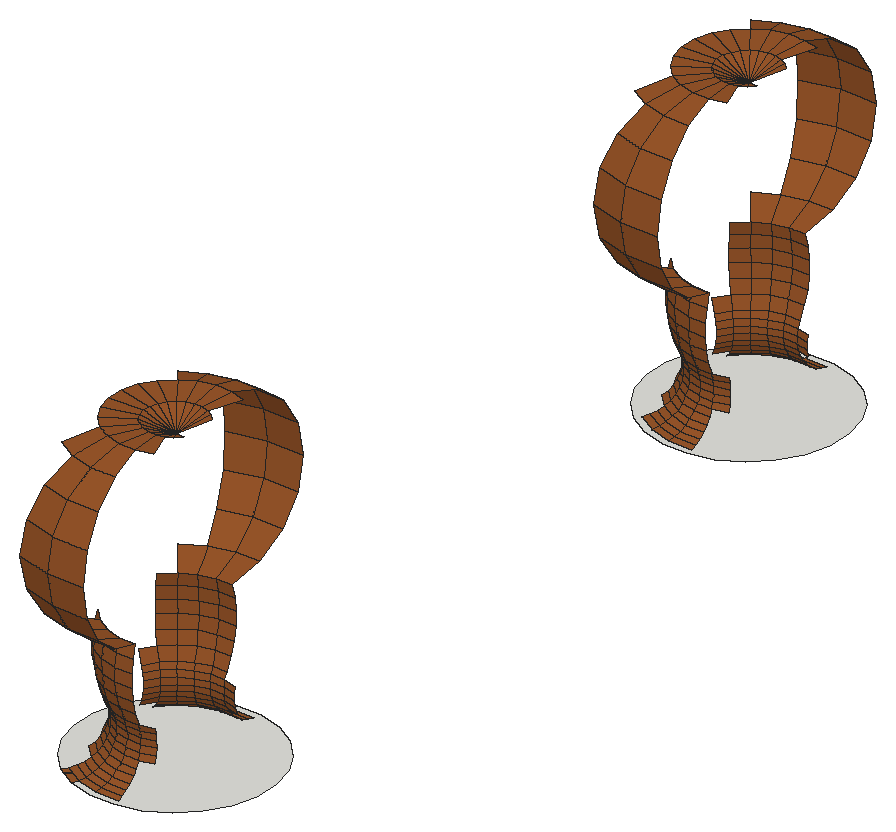
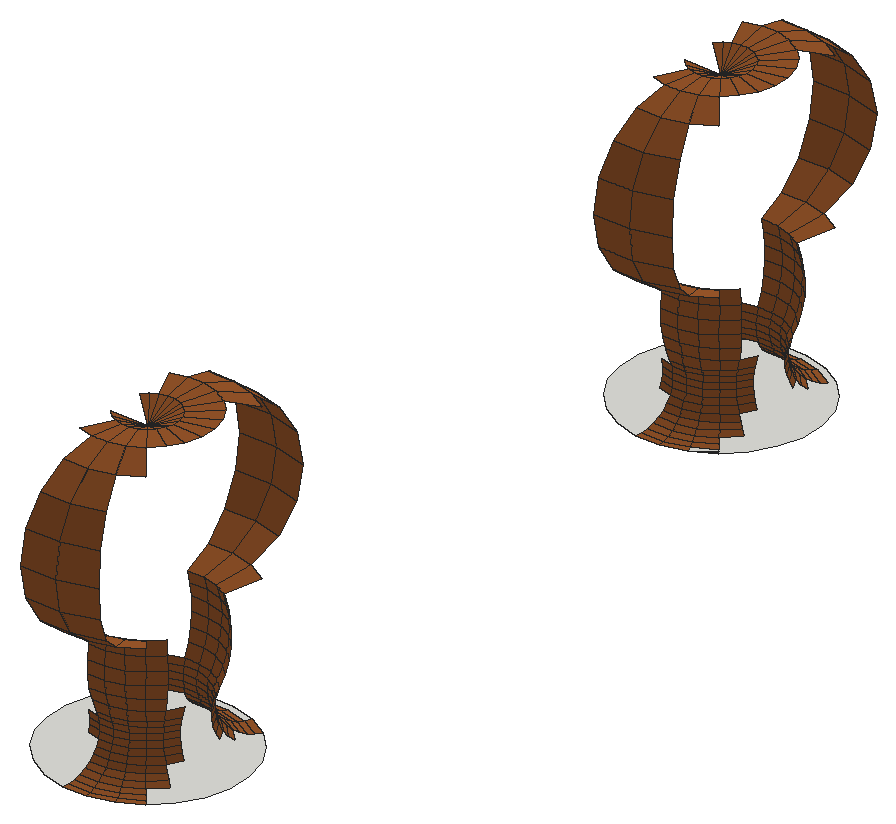
# SketchUp Ruby script. Lengths in inches.
U = 1.inch
M = Sketchup.active_model
def pt(a) = Geom::Point3d.new(a.map { |v| v * U })
def face(e, loops, mat)
  f = e.add_face(loops[0].map { |a| pt(a) })
  loops[1..].each { |l| e.add_face(l.map { |a| pt(a) }).erase! }
  f.material = f.back_material = mat if mat
  f
end
# faces: each face lists its corners as indices into pts; further lists are holes
def faces(e, pts, list, mat = nil) = list.each { |f| face(e, (f[0].is_a?(Array) ? f : [f]).map { |l| l.map { |i| pts[i] } }, mat) }
# xy, xz, yz: faces in a plane at the given z, y or x. An outline is a flat list of corners, or four numbers for a rectangle; further outlines are holes
def ring(l) = l.size == 4 ? [[l[0], l[1]], [l[2], l[1]], [l[2], l[3]], [l[0], l[3]]] : l.each_slice(2).to_a
def flat(e, list, mat, &to3) = list.each { |f| face(e, (f[0].is_a?(Array) ? f : [f]).map { |l| ring(l).map { |u, v| to3.(u, v) } }, mat) }
def xy(e, z, list, mat = nil) = flat(e, list, mat) { |x, y| [x, y, z] }
def xz(e, y, list, mat = nil) = flat(e, list, mat) { |x, z| [x, y, z] }
def yz(e, x, list, mat = nil) = flat(e, list, mat) { |y, z| [x, y, z] }
def lines(e, pts, list) = list.each { |a, b| e.add_line(pt(pts[a]), pt(pts[b])) }
# prism: a flat outline (further loops are holes) pulled along v
def prism(e, loops, v, mat = nil)
  f = face(e, loops, mat); d = Geom::Vector3d.new(v.map { |x| x * U })
  f.pushpull(f.normal.samedirection?(d) ? d.length : -d.length)
end
def box(e, o, s, mat = nil) = prism(e, [[o, [o[0] + s[0], o[1], o[2]], [o[0] + s[0], o[1] + s[1], o[2]], [o[0], o[1] + s[1], o[2]]]], [0, 0, s[2]], mat)
def at(x, y, z, deg = 0) = Geom::Transformation.translation(pt([x, y, z])) * Geom::Transformation.rotation(ORIGIN, Z_AXIS, deg.degrees)
def axes(o, x, y, z) = Geom::Transformation.new([*x, 0, *y, 0, *z, 0, *pt(o).to_a, 1])
def part(name) = M.definitions.add(name)
# library, detail: a bought-in or finely detailed component or shape, given as its bounding box
def library(name, o, s) = part(name).tap { |d| box(d.entities, o, s) }
def detail(e, o, s) = box(e.add_group.entities, o, s)
def put(e, d, t, mat = nil) = e.add_instance(d, t).tap { |i| i.material = mat if mat }
def group(e, t, mat = nil) = e.add_group.tap { |g| g.transformation = t; g.material = mat if mat }.entities
root = M.entities
M.materials.add("[Wood Cherry Original]").color = [152, 86, 42]
xy(root,6,[[160.74,47.97,161.3,47.97,161.84,48.11,162.32,48.39,162.72,48.78,163,49.26,163.15,49.8,163.15,50.36,163.01,50.9,162.73,51.38,162.34,51.78,161.85,52.06,161.32,52.21,160.76,52.21,160.22,52.07,159.73,51.79,159.34,51.4,159.06,50.91,158.91,50.375,158.91,49.82,159.05,49.28,159.33,48.79,159.72,48.4,160.2,48.11],[160.74,64.59,161.3,64.59,161.84,64.73,162.32,65.01,162.72,65.4,163,65.89,163.15,66.42,163.15,66.98,163.01,67.52,162.73,68.01,162.34,68.4,161.85,68.69,161.32,68.83,160.76,68.83,160.22,68.69,159.73,68.41,159.34,68.02,159.06,67.54,158.91,67,158.91,66.44,159.05,65.9,159.33,65.42,159.72,65.02,160.2,64.74]])
xy(root,6,[[160.74,47.97,160.76,48.12,160.26,48.25,160.2,48.11],[160.74,47.97,161.3,47.97,161.28,48.12,160.76,48.12],[160.2,48.11,160.26,48.25,159.8125,48.51,159.72,48.4],[159.82,51.67,160.27,51.93,160.22,52.07,159.73,51.79],[160.27,51.93,160.78,52.06,160.76,52.21,160.22,52.07],
  [160.78,52.06,161.3,52.06,161.32,52.21,160.76,52.21],[160.74,64.59,160.76,64.74,160.26,64.88,160.2,64.74],[160.74,64.59,161.3,64.59,161.28,64.74,160.76,64.74],[160.2,64.74,160.26,64.88,159.8125,65.14,159.72,65.02],[159.82,68.29,160.27,68.55,160.22,68.69,159.73,68.41],
  [160.27,68.55,160.78,68.68,160.76,68.83,160.22,68.69],[160.78,68.68,161.3,68.68,161.32,68.83,160.76,68.83]],"[Wood Cherry Original]")
xz(root,48.59,[[160.83,8.1,161.22,8.4]],"[Wood Cherry Original]")
xz(root,51.28,[[160.875,6.79,161.19,6.94]],"[Wood Cherry Original]")
xz(root,65.52,[[160.87,6.79,161.18,6.94]],"[Wood Cherry Original]")
xz(root,67.9,[[160.875,6.79,161.19,6.94]],"[Wood Cherry Original]")
xz(root,68.21,[[160.84,8.1,161.23,8.4]],"[Wood Cherry Original]")
p = [[160.32,48.39,6.03],[160.26,48.25,6],[160.76,48.12,6],[160.78,48.27,6.03],[161.28,48.12,6],[161.26,48.26,6.03],
  [159.9,48.63,6.03],[159.8125,48.51,6],[160.37,48.52,6.08],[160.8,48.41,6.08],[161.24,48.4,6.08],[159.99,48.75,6.08],
  [160.38,51.66,6.08],[160.33,51.79,6.03],[159.91,51.55,6.03],[160,51.4375,6.08],[160.27,51.93,6],[159.82,51.67,6],
  [160.8125,51.77,6.08],[160.8,51.91,6.03],[160.78,52.06,6],[161.26,51.77,6.08],[161.28,51.91,6.03],[161.3,52.06,6],
  [160.32,65.02,6.03],[160.26,64.88,6],[160.76,64.74,6],[160.78,64.89,6.03],[161.28,64.74,6],[161.26,64.89,6.03],
  [159.9,65.26,6.03],[159.8125,65.14,6],[160.37,65.15,6.08],[160.8,65.03,6.08],[161.24,65.03,6.08],[159.99,65.37,6.08],
  [160.38,68.28,6.08],[160.33,68.41,6.03],[159.91,68.18,6.03],[160,68.0625,6.08],[160.27,68.55,6],[159.82,68.29,6],
  [160.8125,68.4,6.08],[160.8,68.54,6.03],[160.78,68.68,6],[161.26,68.39,6.08],[161.28,68.53,6.03],[161.3,68.68,6],
  [160.42,48.64,6.16],[160.82,48.54,6.16],[161.23,48.53,6.16],[160.07,48.85,6.16],[160.08,51.33,6.16],[159.6875,51.125,6.08],
  [159.79,51.05,6.16],[160.43,51.54,6.16],[160.83,51.64,6.16],[161.24,51.64,6.16],[160.42,65.27,6.16],[160.82,65.16,6.16],
  [161.23,65.16,6.16],[160.07,65.47,6.16],[160.08,67.96,6.16],[159.6875,67.75,6.08],[159.79,67.67,6.16],[160.43,68.16,6.16],
  [160.83,68.27,6.16],[161.24,68.26,6.16],[160.47,48.75,6.25],[160.83,48.65,6.25],[161.21,48.65,6.25],[160.14,48.94,6.25],
  [159.875,49.21,6.25],[159.78,49.14,6.16],[160.15,51.24,6.25],[159.88,50.97,6.25],[160.48,51.43,6.25],[160.84,51.53,6.25],
  [161.22,51.52,6.25],[160.47,65.375,6.25],[160.83,65.27,6.25],[161.21,65.27,6.25],[160.14,65.56,6.25],[159.875,65.83,6.25],
  [159.78,65.76,6.16],[160.15,67.87,6.25],[159.88,67.6,6.25],[160.48,68.05,6.25],[160.84,68.15,6.25],[161.22,68.15,6.25],
  [160.51,48.84,6.37],[160.85,48.75,6.37],[161.2,48.74,6.37],[160.2,49.02,6.37],[159.95,49.27,6.37],[160.21,51.16,6.37],
  [159.96,50.92,6.37],[160.51,51.34,6.37],[160.86,51.43,6.37],[161.21,51.43,6.37],[160.51,65.46,6.37],[160.85,65.37,6.37],
  [161.2,65.37,6.37],[160.2,65.64,6.37],[159.95,65.89,6.37],[160.21,67.79,6.37],[159.96,67.54,6.37],[160.51,67.97,6.37],
  [160.86,68.06,6.37],[161.21,68.05,6.37],[160.53,48.91,6.5],[160.86,48.82,6.5],[161.19,48.82,6.5],[160.25,49.08,6.5],
  [160.01,49.3125,6.5],[159.84,49.6,6.5],[159.78,49.57,6.37],[160.02,50.87,6.5],[159.78,50.61,6.37],[159.85,50.58,6.5],
  [160.25,51.1,6.5],[160.54,51.27,6.5],[160.87,51.36,6.5],[161.2,51.35,6.5],[160.53,65.53,6.5],[160.86,65.44,6.5],
  [161.19,65.44,6.5],[160.25,65.7,6.5],[160.01,65.9375,6.5],[159.84,66.23,6.5],[159.78,66.2,6.37],[160.02,67.49,6.5],
  [159.78,67.24,6.37],[159.85,67.21,6.5],[160.25,67.73,6.5],[160.54,67.9,6.5],[160.87,67.98,6.5],[161.2,67.98,6.5],
  [160.55,48.95,6.64],[160.86,48.87,6.64],[161.18,48.87,6.64],[161.51,48.9,6.5],[161.49,48.95,6.64],[160.28,49.12,6.64],
  [160.05,49.34,6.64],[159.89,49.62,6.64],[160.06,50.84,6.64],[159.9,50.5625,6.64],[160.28,51.0625,6.64],[160.5625,51.22,6.64],
  [160.87,51.3,6.64],[161.5,51.22,6.64],[161.52,51.27,6.5],[161.19,51.3,6.64],[160.55,65.58,6.64],[160.86,65.5,6.64],
  [161.18,65.49,6.64],[161.51,65.53,6.5],[161.49,65.58,6.64],[160.28,65.74,6.64],[160.05,65.97,6.64],[159.89,66.25,6.64],
  [160.06,67.46,6.64],[159.9,67.1875,6.64],[160.28,67.6875,6.64],[160.5625,67.85,6.64],[160.87,67.93,6.64],[161.19,67.93,6.64],
  [160.5625,48.98,6.79],[160.87,48.9,6.79],[161.18,48.9,6.79],[161.48,48.98,6.79],[160.29,49.14,6.79],[160.07,49.36,6.79],
  [159.92,49.63,6.79],[160.08,50.82,6.79],[159.92,50.55,6.79],[160.3,51.04,6.79],[160.57,51.2,6.79],[160.875,51.28,6.79],
  [161.49,51.2,6.79],[161.19,51.28,6.79],[160.5625,65.6,6.79],[160.87,65.52,6.79],[161.18,65.52,6.79],[161.48,65.6,6.79],
  [160.29,65.76,6.79],[160.07,65.98,6.79],[159.92,66.26,6.79],[160.08,67.45,6.79],[159.92,67.18,6.79],[160.3,67.67,6.79],
  [160.57,67.82,6.79],[160.875,67.9,6.79],[161.49,67.82,6.79],[161.5,67.84,6.64],[161.19,67.9,6.79],[160.5625,48.98,6.94],
  [160.87,48.9,6.94],[161.18,48.89,6.94],[161.48,48.97,6.94],[160.29,49.14,6.94],[160.07,49.36,6.94],[159.92,49.63,6.94],
  [160.08,50.82,6.94],[159.92,50.55,6.94],[160.3,51.04,6.94],[160.57,51.2,6.94],[160.875,51.28,6.94],[161.49,51.2,6.94],
  [161.19,51.28,6.94],[160.5625,65.6,6.94],[160.87,65.52,6.94],[161.18,65.52,6.94],[161.48,65.6,6.94],[160.29,65.76,6.94],
  [160.07,65.98,6.94],[159.92,66.26,6.94],[160.08,67.45,6.94],[159.92,67.18,6.94],[160.3,67.67,6.94],[160.57,67.82,6.94],
  [160.875,67.9,6.94],[161.49,67.82,6.94],[161.19,67.9,6.94],[160.55,48.95,7.09],[160.86,48.87,7.09],[161.18,48.87,7.09],
  [161.49,48.95,7.09],[160.28,49.12,7.09],[160.05,49.34,7.09],[159.89,49.62,7.09],[160.06,50.84,7.09],[159.89,50.5625,7.09],
  [160.28,51.06,7.09],[160.5625,51.22,7.09],[160.87,51.31,7.09],[161.5,51.22,7.09],[161.19,51.3,7.09],[160.55,65.58,7.09],
  [160.86,65.49,7.09],[161.18,65.49,7.09],[161.49,65.58,7.09],[160.28,65.74,7.09],[160.05,65.97,7.09],[159.89,66.25,7.09],
  [160.06,67.46,7.09],[159.89,67.1875,7.09],[160.28,67.69,7.09],[160.5625,67.85,7.09],[160.87,67.93,7.09],[161.5,67.85,7.09],
  [161.19,67.93,7.09],[160.53,48.91,7.23],[160.86,48.82,7.23],[161.19,48.82,7.23],[161.51,48.9,7.23],[160.24,49.07,7.23],
  [160.01,49.3125,7.23],[159.84,49.6,7.23],[160.02,50.87,7.23],[159.85,50.58,7.23],[160.25,51.11,7.23],[160.54,51.27,7.23],
  [160.87,51.36,7.23],[161.2,51.36,7.23],[160.53,65.53,7.23],[160.86,65.44,7.23],[161.19,65.44,7.23],[161.51,65.53,7.23],
  [160.24,65.7,7.23],[160.01,65.9375,7.23],[159.84,66.23,7.23],[160.02,67.5,7.23],[159.85,67.21,7.23],[160.25,67.73,7.23],
  [160.54,67.9,7.23],[160.87,67.98,7.23],[161.2,67.98,7.23],[160.49,48.8,7.51],[160.84,48.71,7.51],[161.2,48.71,7.51],
  [160.18,48.99,7.51],[159.92,49.24,7.51],[159.93,50.9375,7.51],[159.74,50.625,7.51],[160.19,51.19,7.51],[160.5,51.375,7.51],
  [160.85,51.47,7.51],[161.22,51.47,7.51],[160.49,65.43,7.51],[160.84,65.33,7.51],[161.2,65.33,7.51],[160.18,65.61,7.51],
  [159.92,65.87,7.51],[159.93,67.5625,7.51],[159.74,67.25,7.51],[160.19,67.82,7.51],[160.5,68,7.51],[160.85,68.09,7.51],
  [161.22,68.09,7.51],[160.46,48.73,7.8],[160.83,48.63,7.8],[161.21,48.63,7.8],[160.13,48.93,7.8],[159.86,49.2,7.8],
  [160.14,51.25,7.8],[159.87,50.98,7.8],[160.47,51.45,7.8],[160.84,51.54,7.8],[161.23,51.54,7.8],[160.46,65.36,7.8],
  [160.83,65.26,7.8],[161.21,65.26,7.8],[160.13,65.55,7.8],[159.86,65.82,7.8],[160.14,67.88,7.8],[159.87,67.61,7.8],
  [160.47,68.07,7.8],[160.84,68.17,7.8],[161.23,68.17,7.8],[160.45,48.7,8.1],[160.83,48.59,8.1],[161.22,48.59,8.1],
  [160.11,48.89,8.1],[159.83,49.17,8.1],[160.12,51.29,8.1],[159.84,51.01,8.1],[160.46,51.48,8.1],[160.84,51.58,8.1],
  [161.23,51.58,8.1],[160.45,65.32,8.1],[160.83,65.22,8.1],[161.22,65.22,8.1],[160.11,65.52,8.1],[159.83,65.8,8.1],
  [160.12,67.91,8.1],[159.84,67.63,8.1],[160.46,68.11,8.1],[160.84,68.21,8.1],[161.23,68.21,8.1],[160.44,48.69,8.4],
  [160.83,48.59,8.4],[160.1,48.89,8.4],[159.83,49.17,8.4],[160.11,51.29,8.4],[159.83,51.01,8.4],[160.46,51.48,8.4],
  [160.84,51.59,8.4],[161.23,51.58,8.4],[160.44,65.32,8.4],[160.83,65.22,8.4],[161.22,65.21,8.4],[160.1,65.52,8.4],
  [159.83,65.8,8.4],[160.11,67.91,8.4],[159.83,67.64,8.4],[160.46,68.11,8.4],[160.84,68.21,8.4],[160.46,48.73,8.7],
  [160.83,48.625,8.7],[161.22,48.59,8.4],[161.22,48.62,8.7],[160.125,48.92,8.7],[159.85,49.19,8.7],[160.13,51.26,8.7],
  [159.86,50.99,8.7],[160.47,51.45,8.7],[160.84,51.55,8.7],[161.23,51.55,8.7],[160.46,65.35,8.7],[160.83,65.25,8.7],
  [161.22,65.25,8.7],[160.125,65.54,8.7],[159.85,65.82,8.7],[160.13,67.89,8.7],[159.86,67.62,8.7],[160.47,68.08,8.7],
  [160.84,68.18,8.7],[161.23,68.17,8.7],[161.23,68.21,8.4],[160.49,48.79,8.99],[160.84,48.69,8.99],[161.21,48.69,8.99],
  [160.17,48.98,8.99],[159.91,49.24,8.99],[160.18,51.21,8.99],[159.92,50.95,8.99],[160.5,51.39,8.99],[160.85,51.48,8.99],
  [161.22,51.48,8.99],[160.49,65.42,8.99],[160.84,65.32,8.99],[161.21,65.32,8.99],[160.17,65.6,8.99],[159.91,65.86,8.99],
  [160.18,67.83,8.99],[159.92,67.57,8.99],[160.5,68.01,8.99],[160.85,68.11,8.99],[161.22,68.1,8.99],[160.21,48.14,9.21],
  [160.74,48,9.21],[161.3,48,9.21],[159.74,48.42,9.21],[160.23,52.04,9.21],[159.75,51.76,9.21],[160.76,52.18,9.21],
  [161.3125,52.18,9.21],[160.21,64.77,9.21],[160.74,64.625,9.21],[161.3,64.62,9.21],[159.74,65.04,9.21],[160.23,68.66,9.21],
  [159.75,68.39,9.21],[160.76,68.8,9.21],[161.3125,68.8,9.21],[159.99,47.61,9.66],[160.67,47.42,9.66],[161.37,47.42,9.66],
  [160.6875,52.75,9.66],[160.01,52.57,9.66],[161.39,52.75,9.66],[159.99,64.23,9.66],[160.67,64.05,9.66],[161.37,64.05,9.66],
  [160.6875,69.38,9.66],[160.01,69.2,9.66],[161.39,69.375,9.66],[159.84,47.26,10.28],[160.62,47.05,10.28],[161.42,47.04,10.28],
  [160.64,53.13,10.28],[159.87,52.93,10.28],[161.44,53.125,10.28],[159.84,63.88,10.28],[160.62,63.67,10.28],[161.42,63.67,10.28],
  [160.64,69.75,10.28],[159.87,69.55,10.28],[161.44,69.75,10.28],[159.79,47.14,11],[160.6,46.92,11],[161.43,46.91,11],
  [160.62,53.26,11],[159.81,53.05,11],[161.46,53.26,11],[159.79,63.76,11],[160.6,63.54,11],[161.43,63.54,11],
  [160.62,69.89,11],[159.81,69.67,11],[161.46,69.88,11],[159.84,47.26,11.72],[160.62,47.05,11.72],[161.42,47.04,11.72],
  [160.64,53.13,11.72],[159.87,52.93,11.72],[161.44,53.125,11.72],[159.84,63.88,11.72],[160.62,63.67,11.72],[161.42,63.67,11.72],
  [160.64,69.75,11.72],[159.87,69.55,11.72],[161.44,69.75,11.72],[159.99,47.61,12.34],[160.67,47.42,12.34],[161.37,47.42,12.34],
  [160.6875,52.75,12.34],[160.01,52.57,12.34],[161.39,52.75,12.34],[159.99,64.23,12.34],[160.67,64.05,12.34],[161.37,64.05,12.34],
  [160.6875,69.38,12.34],[160.01,69.2,12.34],[161.39,69.375,12.34],[160.21,48.14,12.79],[160.74,48,12.79],[161.3,48,12.79],
  [160.76,52.18,12.79],[160.23,52.04,12.79],[161.3125,52.18,12.79],[160.21,64.77,12.79],[160.74,64.625,12.79],[161.3,64.62,12.79],
  [160.76,68.8,12.79],[160.23,68.66,12.79],[161.3125,68.8,12.79],[161.03,50.09,12.67],[160.77,49.47,12.97],[160.9375,49.42,12.97],
  [161.11,49.42,12.97],[161.28,49.47,12.97],[160.62,49.56,12.97],[161.43,49.55,12.97],[160.49,49.68,12.97],[161.56,49.68,12.97],
  [160.41,49.83,12.97],[160.36,50,12.97],[160.36,50.18,12.97],[160.41,50.35,12.97],[160.5,50.5,12.97],[160.62,50.62,12.97],
  [160.77,50.71,12.97],[160.94,50.75,12.97],[161.12,50.75,12.97],[161.29,50.71,12.97],[161.4375,50.62,12.97],[161.5625,50.49,12.97],
  [161.03,66.71,12.67],[160.77,66.09,12.97],[160.9375,66.05,12.97],[161.11,66.05,12.97],[161.28,66.09,12.97],[160.62,66.18,12.97],
  [161.43,66.18,12.97],[160.49,66.31,12.97],[161.56,66.3,12.97],[160.41,66.46,12.97],[160.36,66.63,12.97],[160.36,66.8,12.97],
  [160.41,66.97,12.97],[160.5,67.12,12.97],[160.62,67.25,12.97],[160.77,67.33,12.97],[160.94,67.38,12.97],[161.12,67.38,12.97],
  [161.29,67.33,12.97],[161.4375,67.24,12.97],[161.5625,67.12,12.97],[160.49,48.79,13.01],[160.84,48.69,13.01],[161.21,48.69,13.01],
  [160.17,48.98,13.01],[159.74,48.42,12.79],[160.5,51.39,13.01],[159.75,51.76,12.79],[160.18,51.21,13.01],[160.85,51.48,13.01],
  [161.22,51.48,13.01],[160.49,65.42,13.01],[160.84,65.32,13.01],[161.21,65.32,13.01],[160.17,65.6,13.01],[159.74,65.04,12.79],
  [160.5,68.01,13.01],[159.75,68.39,12.79],[160.18,67.83,13.01],[160.85,68.11,13.01],[161.22,68.1,13.01],[161.5625,48.79,13.01],
  [159.91,49.24,13.01],[159.73,49.55,13.01],[159.63,49.91,13.01],[159.64,50.28,13.01],[159.73,50.63,13.01],[159.92,50.95,13.01],
  [161.57,51.38,13.01],[161.5625,65.41,13.01],[159.91,65.86,13.01],[159.73,66.18,13.01],[159.63,66.53,13.01],[159.64,66.9,13.01],
  [159.73,67.26,13.01],[159.92,67.57,13.01],[161.57,68.01,13.01]]
faces(root,p,[[0,1,2,3],[3,2,4,5],[6,7,1,0],[8,0,3,9],[9,3,5,10],[11,6,0,8],[12,13,14,15],[13,16,17,14],
  [18,19,13,12],[19,20,16,13],[21,22,19,18],[22,23,20,19],[24,25,26,27],[27,26,28,29],[30,31,25,24],[32,24,27,33],
  [33,27,29,34],[35,30,24,32],[36,37,38,39],[37,40,41,38],[42,43,37,36],[43,44,40,37],[45,46,43,42],[46,47,44,43],
  [48,8,9,49],[49,9,10,50],[51,11,8,48],[52,15,53,54],[55,12,15,52],[56,18,12,55],[57,21,18,56],[58,32,33,59],
  [59,33,34,60],[61,35,32,58],[62,39,63,64],[65,36,39,62],[66,42,36,65],[67,45,42,66],[68,48,49,69],[69,49,50,70],
  [71,51,48,68],[72,73,51,71],[74,52,54,75],[76,55,52,74],[77,56,55,76],[78,57,56,77],[79,58,59,80],[80,59,60,81],
  [82,61,58,79],[83,84,61,82],[85,62,64,86],[87,65,62,85],[88,66,65,87],[89,67,66,88],[90,68,69,91],[91,69,70,92],
  [93,71,68,90],[94,72,71,93],[95,74,75,96],[97,76,74,95],[98,77,76,97],[99,78,77,98],[100,79,80,101],[101,80,81,102],
  [103,82,79,100],[104,83,82,103],[105,85,86,106],[107,87,85,105],[108,88,87,107],[109,89,88,108],[110,90,91,111],[111,91,92,112],
  [113,93,90,110],[114,94,93,113],[115,116,94,114],[117,96,118,119],[120,95,96,117],[121,97,95,120],[122,98,97,121],[123,99,98,122],
  [124,100,101,125],[125,101,102,126],[127,103,100,124],[128,104,103,127],[129,130,104,128],[131,106,132,133],[134,105,106,131],[135,107,105,134],
  [136,108,107,135],[137,109,108,136],[138,110,111,139],[139,111,112,140],[140,112,141,142],[143,113,110,138],[144,114,113,143],[145,115,114,144],
  [146,117,119,147],[148,120,117,146],[149,121,120,148],[150,122,121,149],[151,152,123,153],[153,123,122,150],[154,124,125,155],[155,125,126,156],
  [156,126,157,158],[159,127,124,154],[160,128,127,159],[161,129,128,160],[162,131,133,163],[164,134,131,162],[165,135,134,164],[166,136,135,165],
  [167,137,136,166],[168,138,139,169],[169,139,140,170],[170,140,142,171],[172,143,138,168],[173,144,143,172],[174,145,144,173],[175,146,147,176],
  [177,148,146,175],[178,149,148,177],[179,150,149,178],[180,151,153,181],[181,153,150,179],[182,154,155,183],[183,155,156,184],[184,156,158,185],
  [186,159,154,182],[187,160,159,186],[188,161,160,187],[189,162,163,190],[191,164,162,189],[192,165,164,191],[193,166,165,192],[194,195,167,196],
  [196,167,166,193],[197,168,169,198],[198,169,170,199],[199,170,171,200],[201,172,168,197],[202,173,172,201],[203,174,173,202],[204,175,176,205],
  [206,177,175,204],[207,178,177,206],[208,179,178,207],[209,180,181,210],[211,182,183,212],[213,184,185,214],[215,186,182,211],[216,187,186,215],
  [217,188,187,216],[218,189,190,219],[220,191,189,218],[221,192,191,220],[222,193,192,221],[223,194,196,224],[225,197,198,226],[226,198,199,227],
  [227,199,200,228],[229,201,197,225],[230,202,201,229],[231,203,202,230],[232,204,205,233],[234,206,204,232],[235,207,206,234],[236,208,207,235],
  [237,209,210,238],[238,210,208,236],[239,211,212,240],[240,212,213,241],[241,213,214,242],[243,215,211,239],[244,216,215,243],[245,217,216,244],
  [246,218,219,247],[248,220,218,246],[249,221,220,248],[250,222,221,249],[251,223,224,252],[252,224,222,250],[253,225,226,254],[254,226,227,255],
  [255,227,228,256],[257,229,225,253],[258,230,229,257],[259,231,230,258],[260,232,233,261],[262,234,232,260],[263,235,234,262],[264,236,235,263],
  [265,238,236,264],[266,239,240,267],[267,240,241,268],[268,241,242,269],[270,243,239,266],[271,244,243,270],[272,245,244,271],[273,246,247,274],
  [275,248,246,273],[276,249,248,275],[277,250,249,276],[278,252,250,277],[279,253,254,280],[280,254,255,281],[282,257,253,279],[283,258,257,282],
  [284,260,261,285],[286,262,260,284],[287,263,262,286],[288,264,263,287],[289,265,264,288],[290,266,267,291],[291,267,268,292],[293,270,266,290],
  [294,271,270,293],[295,273,274,296],[297,275,273,295],[298,276,275,297],[299,277,276,298],[300,278,277,299],[301,279,280,302],[302,280,281,303],
  [304,282,279,301],[305,283,282,304],[306,286,284,307],[308,287,286,306],[309,288,287,308],[310,289,288,309],[311,290,291,312],[312,291,292,313],
  [314,293,290,311],[315,294,293,314],[316,297,295,317],[318,298,297,316],[319,299,298,318],[320,300,299,319],[321,301,302,322],[322,302,303,323],
  [324,304,301,321],[325,305,304,324],[326,306,307,327],[328,308,306,326],[329,309,308,328],[330,310,309,329],[331,311,312,332],[332,312,313,333],
  [334,314,311,331],[335,315,314,334],[336,316,317,337],[338,318,316,336],[339,319,318,338],[340,320,319,339],[341,321,322,342],[343,324,321,341],
  [344,325,324,343],[345,326,327,346],[347,328,326,345],[348,329,328,347],[349,330,329,348],[350,331,332,351],[351,332,333,352],[353,334,331,350],
  [354,335,334,353],[355,336,337,356],[357,338,336,355],[358,339,338,357],[359,341,342,360],[360,342,361,362],[363,343,341,359],[364,344,343,363],
  [365,345,346,366],[367,347,345,365],[368,348,347,367],[369,349,348,368],[370,350,351,371],[371,351,352,372],[373,353,350,370],[374,354,353,373],
  [375,355,356,376],[377,357,355,375],[378,358,357,377],[379,380,358,378],[381,359,360,382],[382,360,362,383],[384,363,359,381],[385,364,363,384],
  [386,365,366,387],[388,367,365,386],[389,368,367,388],[390,369,368,389],[391,370,371,392],[392,371,372,393],[394,373,370,391],[395,374,373,394],
  [396,375,376,397],[398,377,375,396],[399,378,377,398],[400,379,378,399],[401,381,382,402],[402,382,383,403],[404,384,381,401],[405,388,386,406],
  [407,389,388,405],[408,390,389,407],[409,391,392,410],[410,392,393,411],[412,394,391,409],[413,398,396,414],[415,399,398,413],[416,400,399,415],
  [417,401,402,418],[418,402,403,419],[420,407,405,421],[422,408,407,420],[423,409,410,424],[424,410,411,425],[426,415,413,427],[428,416,415,426],
  [429,417,418,430],[430,418,419,431],[432,420,421,433],[434,422,420,432],[435,423,424,436],[436,424,425,437],[438,426,427,439],[440,428,426,438],
  [441,429,430,442],[442,430,431,443],[444,432,433,445],[446,434,432,444],[447,435,436,448],[448,436,437,449],[450,438,439,451],[452,440,438,450],
  [453,441,442,454],[454,442,443,455],[456,444,445,457],[458,446,444,456],[459,447,448,460],[460,448,449,461],[462,450,451,463],[464,452,450,462],
  [465,453,454,466],[466,454,455,467],[468,456,457,469],[470,458,456,468],[471,459,460,472],[472,460,461,473],[474,462,463,475],[476,464,462,474],
  [477,465,466,478],[478,466,467,479],[480,468,469,481],[482,470,468,480],[483,471,472,484],[484,472,473,485],[486,474,475,487],[488,476,474,486],
  [489,490,491],[489,491,492],[489,492,493],[489,494,490],[489,493,495],[489,496,494],[489,495,497],[489,498,496],
  [489,499,498],[489,500,499],[489,501,500],[489,502,501],[489,503,502],[489,504,503],[489,505,504],[489,506,505],
  [489,507,506],[489,508,507],[489,509,508],[510,511,512],[510,512,513],[510,513,514],[510,515,511],[510,514,516],
  [510,517,515],[510,516,518],[510,519,517],[510,520,519],[510,521,520],[510,522,521],[510,523,522],[510,524,523],
  [510,525,524],[510,526,525],[510,527,526],[510,528,527],[510,529,528],[510,530,529],[531,477,478,532],[532,478,479,533],
  [534,535,477,531],[536,481,537,538],[539,480,481,536],[540,482,480,539],[541,483,484,542],[542,484,485,543],[544,545,483,541],[546,487,547,548],
  [549,486,487,546],[550,488,486,549],[490,531,532,491],[491,532,533,492],[492,533,551,493],[494,534,531,490],[496,552,534,494],[498,553,552,496],
  [499,554,553,498],[500,555,554,499],[501,556,555,500],[502,557,556,501],[503,538,557,502],[504,536,538,503],[505,539,536,504],[507,558,540,506],
  [506,540,539,505],[511,541,542,512],[512,542,543,513],[513,543,559,514],[515,544,541,511],[517,560,544,515],[519,561,560,517],[520,562,561,519],
  [521,563,562,520],[522,564,563,521],[523,565,564,522],[524,548,565,523],[525,546,548,524],[526,549,546,525],[528,566,550,527],[527,550,549,526]],"[Wood Cherry Original]")
